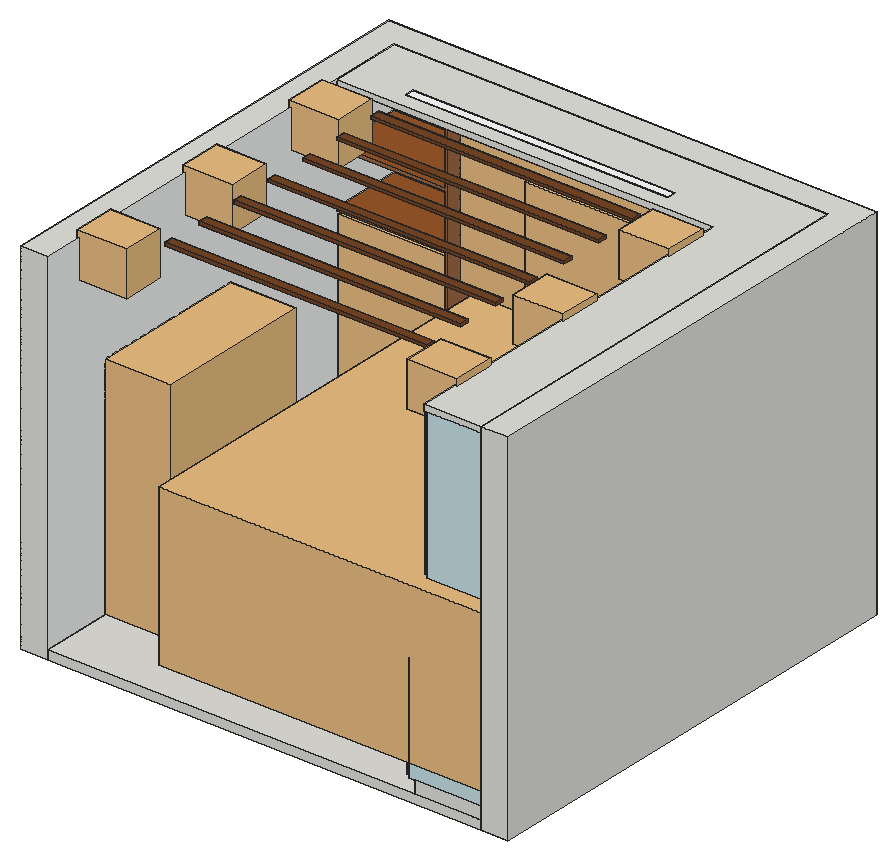
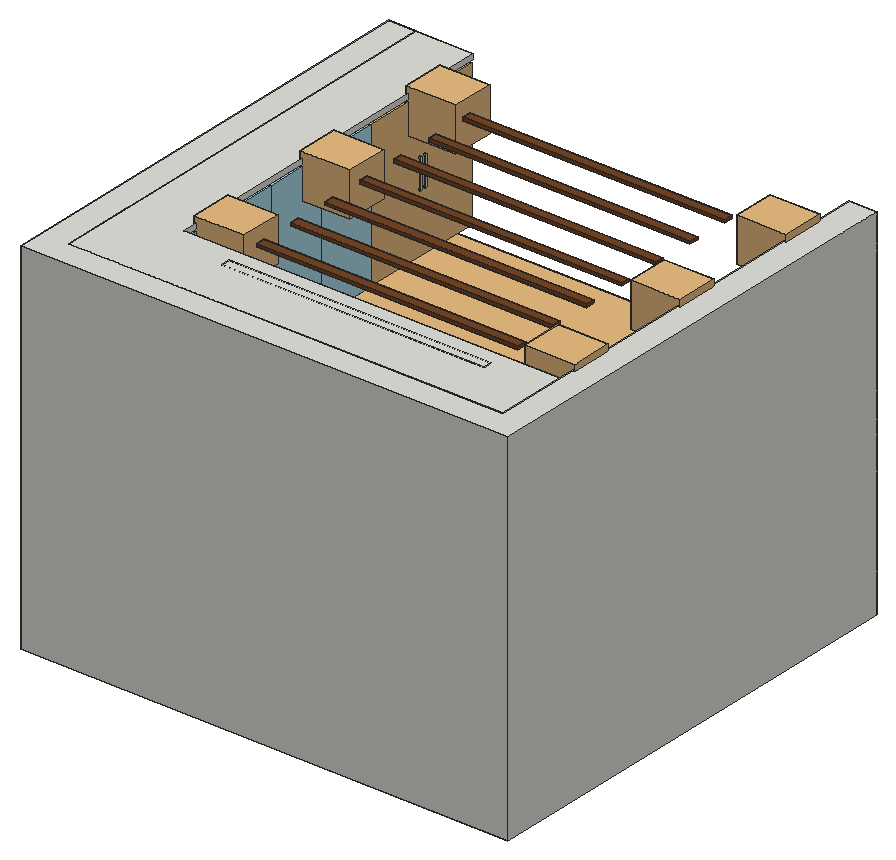
# SketchUp Ruby script. Lengths in inches.
U = 1.inch
M = Sketchup.active_model
def pt(a) = Geom::Point3d.new(a.map { |v| v * U })
def face(e, loops, mat)
  f = e.add_face(loops[0].map { |a| pt(a) })
  loops[1..].each { |l| e.add_face(l.map { |a| pt(a) }).erase! }
  f.material = f.back_material = mat if mat
  f
end
# faces: each face lists its corners as indices into pts; further lists are holes
def faces(e, pts, list, mat = nil) = list.each { |f| face(e, (f[0].is_a?(Array) ? f : [f]).map { |l| l.map { |i| pts[i] } }, mat) }
# xy, xz, yz: faces in a plane at the given z, y or x. An outline is a flat list of corners, or four numbers for a rectangle; further outlines are holes
def ring(l) = l.size == 4 ? [[l[0], l[1]], [l[2], l[1]], [l[2], l[3]], [l[0], l[3]]] : l.each_slice(2).to_a
def flat(e, list, mat, &to3) = list.each { |f| face(e, (f[0].is_a?(Array) ? f : [f]).map { |l| ring(l).map { |u, v| to3.(u, v) } }, mat) }
def xy(e, z, list, mat = nil) = flat(e, list, mat) { |x, y| [x, y, z] }
def xz(e, y, list, mat = nil) = flat(e, list, mat) { |x, z| [x, y, z] }
def yz(e, x, list, mat = nil) = flat(e, list, mat) { |y, z| [x, y, z] }
def lines(e, pts, list) = list.each { |a, b| e.add_line(pt(pts[a]), pt(pts[b])) }
# prism: a flat outline (further loops are holes) pulled along v
def prism(e, loops, v, mat = nil)
  f = face(e, loops, mat); d = Geom::Vector3d.new(v.map { |x| x * U })
  f.pushpull(f.normal.samedirection?(d) ? d.length : -d.length)
end
def box(e, o, s, mat = nil) = prism(e, [[o, [o[0] + s[0], o[1], o[2]], [o[0] + s[0], o[1] + s[1], o[2]], [o[0], o[1] + s[1], o[2]]]], [0, 0, s[2]], mat)
def at(x, y, z, deg = 0) = Geom::Transformation.translation(pt([x, y, z])) * Geom::Transformation.rotation(ORIGIN, Z_AXIS, deg.degrees)
def axes(o, x, y, z) = Geom::Transformation.new([*x, 0, *y, 0, *z, 0, *pt(o).to_a, 1])
def part(name) = M.definitions.add(name)
# library, detail: a bought-in or finely detailed component or shape, given as its bounding box
def library(name, o, s) = part(name).tap { |d| box(d.entities, o, s) }
def detail(e, o, s) = box(e.add_group.entities, o, s)
def put(e, d, t, mat = nil) = e.add_instance(d, t).tap { |i| i.material = mat if mat }
def group(e, t, mat = nil) = e.add_group.tap { |g| g.transformation = t; g.material = mat if mat }.entities
root = M.entities
M.materials.add("0184 AP 7363 HIGH SPIRITS").color = [199, 226, 231]
M.materials.add("0441 AP 9210 SOFT BLUE").color = [171, 218, 233]
M.materials.add("Dado").color = [252, 229, 201]
M.materials.add("W146Z460B75_NILAYA CITY GLAM 32611 ROLL B75").color = [241, 242, 243]
M.materials.add("[Carrera Marble]").color = [207, 207, 207]
M.materials.add("[Color M00]").color = [255, 255, 255]
M.materials.add("[Marble Carrara Gold Floor Tile]").color = [225, 223, 217]
M.materials.add("[Stone Marble]").color = [143, 138, 136]
M.materials.add("[Translucent Glass Blue]").color = [154, 179, 222]
M.materials["[Translucent Glass Blue]"].alpha = 0.5
M.materials.add("[Wood Cherry Original]").color = [152, 86, 42]
M.materials.add("[Wood Floor Parquet]").color = [160, 112, 68]
M.materials.add("[Wood Veneer 01]").color = [160, 105, 68]
M.materials.add("[Wood Veneer 01]1").color = [120, 70, 37]
c1 = library("Group\#91",[0,-4,0],[52,76,21.875])
c2 = library("French door refrigerator",[0,0,0],[35.5,29.25,69.5])
c3 = part("1")
detail(c3.entities,[-0.45,-1,-0.3],[35.9,1,11.43])
c4 = part("2")
box(c4.entities,[-1,-0.3,-0.3],[1,40.1,17.1])
c5 = library("Group\#27",[-1,-0.3,-0.3],[1,40.1,34.6])
c6 = library("Group\#7",[0,0,-31.45],[107,144,53.06])
c7 = part("3")
box(c7.entities,[-20,0,0],[20,41,0.39])
c8 = part("POI-E1497-320-1917\#1")
xy(c8.entities,0,[[0,0,0.29,0.83],[7.21,0,7.5,0.83]])
xy(c8.entities,0.64,[[0.29,0.21,7.21,0.62]])
xy(c8.entities,0.875,[[0,0.21,7.5,0.62]])
xz(c8.entities,0.21,[[0,0.64,7.5,0.875]])
xz(c8.entities,0.62,[[0,0.64,7.5,0.875]])
yz(c8.entities,0,[[0,0,0.21,0.64,0.21,0.875,0.62,0.875,0.62,0.64,0.83,0]])
yz(c8.entities,0.29,[[0,0,0.83,0,0.62,0.64,0.21,0.64]])
yz(c8.entities,7.21,[[0,0,0.21,0.64,0.62,0.64,0.83,0]])
yz(c8.entities,7.5,[[0,0,0.83,0,0.62,0.64,0.62,0.875,0.21,0.875,0.21,0.64]])
p = [[0,0.21,0.64],[0,0,0],[0.29,0,0],[0.29,0.21,0.64],[7.21,0.21,0.64],[7.21,0,0],
  [7.5,0,0],[7.5,0.21,0.64],[0,0.83,0],[0,0.62,0.64],[0.29,0.62,0.64],[0.29,0.83,0],
  [7.5,0.83,0],[7.5,0.62,0.64],[7.21,0.62,0.64],[7.21,0.83,0]]
faces(c8.entities,p,[[0,1,2,3],[4,5,6,7],[8,9,10,11],[12,13,14,15]])
c9 = library("13",[0,-0.4,-0.4],[1.79,16.97,40.8])
c10 = library("kitchen utensil",[-39.88,-27.4,0],[79.77,28.4,32.96])
c11 = library("Group\#26",[0,0,0],[28.9375,18.36,1.53])
c12 = library("Cookware hanging rail",[-2.09,-19.1875,0],[25.71,19.1875,6.07])
c13 = library("switch board",[0,0,0],[0.88,10.49,5.27])
c14 = part("6")
box(c14.entities,[-1,20.47,-0.3],[1,20.66,48.01])
box(c14.entities,[-1,-0.3,-0.3],[1,20.67,48.01])
p = [[0,20.47,47.71],[0,20.37,47.71]]
lines(c14.entities,p,[[0,1]])
c15 = part("7")
prism(c15.entities,[[[0,0.25,0],[0,0.5,0],[0.88,0.5,0],[0.88,0.25,0],[0.86,0.22,0],[0.84,0.19,0],[0.81,0.17,0],[0.79,0.14,0],[0.76,0.12,0],[0.74,0.1,0],[0.71,0.08,0],[0.68,0.06,0],[0.64,0.04,0],[0.61,0.03,0],[0.58,0.02,0],[0.54,0.01,0],[0.51,0,0],[0.47,0,0],[0.4375,0,0],[0.4,0,0],[0.37,0,0],[0.33,0.01,0],[0.3,0.02,0],[0.27,0.03,0],[0.23,0.04,0],[0.2,0.06,0],[0.17,0.08,0],[0.14,0.1,0],[0.11,0.12,0],[0.09,0.14,0],[0.0625,0.17,0],[0.04,0.19,0],[0.02,0.22,0]]],[0,0,47.41])
c16 = library("Group\#12",[0,0,0],[107,19,49.41])
c17 = library("Group\#10",[-1,-0.3,-0.3],[1,40.1,34.6])
c18 = library("Rangemaaster flat hood",[-3.82,0.71,0],[43.23,19.01,40.35])
c19 = part("Group156\#1")
p = [[0,0,0],[0,0,-10.12],[-5.02,0,-10.12],[32.7,-0.05,0],[-32.7,-0.05,0],[32.7,0.05,0],
  [32.7,0,0],[-32.7,0.05,0],[5.02,0,-10.12],[-32.7,0,0],[0,0,-16.375]]
lines(c19.entities,p,[[0,1],[1,2],[3,4],[5,6],[7,5],[1,8],[9,0],[0,6],[8,10],[4,9],[6,3],[2,10],
  [9,7]])
c20 = part("Rectangle Light")
put(c20.entities,c19,at(0,0,0))
c21 = part("5")
xy(c21.entities,-0.61,[[-17,0.0625,-16,40.83]])
xy(c21.entities,-0.44,[[-16.3125,0.0625,-16,40.83]])
xy(c21.entities,-0.11,[[-16.3125,0.0625,-16,40.83]])
xy(c21.entities,0,[[-16,0,0,40.83]],"[Translucent Glass Blue]")
xy(c21.entities,0.39,[[-17,0.0625,-16,40.83]])
xy(c21.entities,0.39,[[-16,0,0,40.83]],"[Translucent Glass Blue]")
xz(c21.entities,0,[[-16,0,0,0.39]],"[Translucent Glass Blue]")
xz(c21.entities,0.0625,[[-17,-0.61,-16,-0.61,-16,-0.44,-16.3125,-0.44,-16.3125,-0.11,-16,-0.11,-16,0.39,-17,0.39]])
xz(c21.entities,40.83,[[-16,0,0,0.39]],"[Translucent Glass Blue]")
yz(c21.entities,-17,[[0.0625,-0.61,40.83,0.39]])
yz(c21.entities,-16.3125,[[0.0625,-0.44,40.83,-0.11]])
yz(c21.entities,-16,[[0.0625,-0.61,40.83,-0.44],[0.0625,-0.11,40.83,0],[0.0625,0,40.83,0.39]])
yz(c21.entities,-16,[[0,0,0.0625,0.39]],"[Translucent Glass Blue]")
yz(c21.entities,0,[[0,0,40.83,0.39]],"[Translucent Glass Blue]")
put(c21.entities,c20,axes([-16.03,20.45,-0.19],[0,0.62341,0],[-0.20108,0,-0.97958],[-0.97958,0,0.20108]))
g1 = group(c21.entities,at(-16.3125,0.0625,-0.27))
box(g1,[0,0,0],[0.25,40.77,0.17])
c22 = library("9",[-6.9,-3.96,-12.62],[16.56,13.95,14.65])
c23 = part("11")
box(c23.entities,[-1,0,-1],[87,3,1])
xy(root,0,[[0,0,0,153,162,153,162,0,153,0,153,144,9,144,9,0]])
xy(root,3,[[131,0,153,128],[9,120,9,144,153,144,153,128,46,128,46,120]])
xy(root,7,[[131,0,153,128],[9,120,45,144],[45,120,46,144],[46,128,153,144]])
xy(root,60.16,[[153,109.21,153.5,119.7]],"[Carrera Marble]")
xy(root,65.43,[[153,109.21,153.5,119.7]],"[Carrera Marble]")
xy(root,81,[[9,120,45,143.92]],"[Wood Cherry Original]")
xy(root,82,[[9,120,45,143.92]],"[Wood Cherry Original]")
xy(root,99.5,[[9,120,45,143.92]],"[Wood Cherry Original]")
xy(root,100.5,[[9,120,45,143.92]],"[Wood Cherry Original]")
xy(root,118.03,[[134,0,153,120],[9,120,45,143.92],[45,120,46,144],[46,120,153,144]])
xy(root,120,[[0,0,9,0,9,144,153,144,153,0,162,0,162,153,0,153],[134,0,153,0,153,144,9,144,9,120,134,120]])
xz(root,0,[[0,0,9,120],[153,0,162,120],[131,3,153,7],[134,118.03,153,120]])
xz(root,109.21,[[153,60.16,153.5,65.43]],"[Carrera Marble]")
xz(root,119.7,[[153,60.16,153.5,65.43]],"[Carrera Marble]")
xz(root,120,[[9,118.03,134,120]])
xz(root,120,[[9,3,46,7]],"[Carrera Marble]")
xz(root,120,[[45,7,46,7,46,118.03,45,118.03,45,100.5,9,100.5,9,99.5,45,99.5,45,82,9,82,9,81,45,81]],"[Wood Veneer 01]")
xz(root,128,[[131,3,153,7]])
xz(root,128,[[46,3,131,7]],"[Carrera Marble]")
xz(root,143.92,[[9,81,45,82],[9,99.5,45,100.5]],"[Wood Cherry Original]")
xz(root,143.92,[[9,82,45,99.5],[9,100.5,45,118.03]],"[Wood Veneer 01]")
xz(root,144,[[9,0,153,0,153,45,46,45,46,68.62,62.64,68.62,62.64,72.3125,118.36,72.3125,118.36,68.62,153,68.62,153,120,9,120],[9,3,153,7],[45,7,46,7,46,118.03,45,118.03,45,98.5,9,98.5,9,97.5,45,97.5]])
xz(root,144,[[46,45,153,45,153,68.62,118.36,68.62,118.36,72.3125,62.64,72.3125,62.64,68.62,46,68.62]],"[Carrera Marble]")
xz(root,144,[[9,98.5,45,118.03]],"[Wood Veneer 01]")
xz(root,153,[[0,0,162,120]])
yz(root,0,[[0,0,153,120]])
yz(root,9,[[120,3,144,7],[120,81,143.92,82],[143.92,97.5,144,98.5],[120,99.5,143.92,100.5],[120,118.03,144,120]])
yz(root,9,[[0,0,144,120]],"W146Z460B75_NILAYA CITY GLAM 32611 ROLL B75")
yz(root,9,[[143.92,76,144,97.5],[143.92,98.5,144,118.03]],"[Wood Veneer 01]")
yz(root,45,[[120,7,120,81,143.92,81,143.92,76,144,76,144,7]],"[Wood Cherry Original]")
yz(root,45,[[143.92,76,144,97.5],[120,82,143.92,99.5],[143.92,98.5,144,118.03],[120,100.5,143.92,118.03]],"[Wood Veneer 01]")
yz(root,46,[[120,3,128,7]],"[Carrera Marble]")
yz(root,46,[[120,7,144,118.03]],"[Wood Veneer 01]")
yz(root,131,[[0,3,128,7]],"[Carrera Marble]")
yz(root,134,[[0,118.03,120,120]])
yz(root,153,[[0,0,144,45],[0,3,128,7],[128,3,144,7],[0,68.62,144,120],[120,118.03,144,120]])
yz(root,153,[[[0,45,144,68.62],[109.21,60.16,119.7,65.43]]],"[Carrera Marble]")
yz(root,153.5,[[109.21,60.16,119.7,65.43]],"[Carrera Marble]")
yz(root,162,[[0,0,153,120]])
p = [[153,144,45],[153,144,70.59],[9,144,76],[9,144,7]]
lines(root,p,[[0,1],[2,3]])
g2 = group(root,at(9,0,0))
xy(g2,0,[[0,0,144,144]])
xy(g2,3,[[122,0,144,0,144,144,0,144,0,120,37,120,37,128,122,128]])
xy(g2,3,[[0,0,122,0,122,128,37,128,37,120,0,120]],"[Marble Carrara Gold Floor Tile]")
xz(g2,0,[[0,0,144,3]])
xz(g2,144,[[0,0,144,3]])
yz(g2,0,[[0,0,144,3]])
yz(g2,144,[[0,0,144,3]])
put(root,c1,axes([9,24,7],[0,1,0],[0,0,1],[1,0,0]))
g3 = group(root,at(46,144,7),"0184 AP 7363 HIGH SPIRITS")
xy(g3,0,[[0,-20,83,0]])
xy(g3,1,[[1,-20,36,-1],[37,-20,67,-1],[68,-20,80,-1]])
xy(g3,11.83,[[1,-20,36,-1]])
xy(g3,12.83,[[1,-20,36,-1]])
xy(g3,17.5,[[68,-20,80,-1]])
xy(g3,18.5,[[68,-20,80,-1]])
xy(g3,23.17,[[1,-20,36,-1]])
xy(g3,24.17,[[1,-20,36,-1]])
xy(g3,35,[[1,-20,36,-1],[37,-20,67,-1],[68,-20,80,-1]])
xy(g3,36,[[0,-20,83,0]])
xz(g3,-20,[[[0,0,83,36],[37,1,67,35],[1,1,36,11.83],[1,24.17,36,35],[1,12.83,36,23.17],[68,18.5,80,35],[68,1,80,17.5]]])
xz(g3,-1,[[1,1,36,11.83],[37,1,67,35],[68,1,80,17.5],[1,12.83,36,23.17],[68,18.5,80,35],
  [1,24.17,36,35]])
xz(g3,0,[[0,0,83,36]])
yz(g3,0,[[-20,0,0,36]])
yz(g3,1,[[-20,1,-1,11.83],[-20,12.83,-1,23.17],[-20,24.17,-1,35]])
yz(g3,36,[[-20,1,-1,11.83],[-20,12.83,-1,23.17],[-20,24.17,-1,35]])
yz(g3,37,[[-20,1,-1,35]])
yz(g3,67,[[-20,1,-1,35]])
yz(g3,68,[[-20,1,-1,17.5],[-20,18.5,-1,35]])
yz(g3,80,[[-20,1,-1,17.5],[-20,18.5,-1,35]])
yz(g3,83,[[-20,0,0,36]])
g4 = group(root,at(153,0,7),"0184 AP 7363 HIGH SPIRITS")
xy(g4,0,[[-24,0,0,128],[-24,128,0,144]])
xy(g4,1,[[-24,1,-2.77,42],[-24,43,-2.77,82.5],[-24,83.5,-2.77,83.5,-2.77,143,-23.08,143,-23.08,122,-24,122]])
xy(g4,11.83,[[-23.08,83.5,-2.77,143]])
xy(g4,12.83,[[-23.08,83.5,-2.77,143]])
xy(g4,17.5,[[-24,43,-2.77,82.5]])
xy(g4,18.5,[[-24,43,-2.77,82.5]])
xy(g4,23.17,[[-23.08,83.5,-2.77,143]])
xy(g4,24.17,[[-23.08,83.5,-2.77,143]])
xy(g4,30.3125,[[-22,43,-5.47,43,-5.47,79.65,-22,79.57]])
xy(g4,33.0625,[[-22,42.27,-5.47,42.35,-5.47,43,-22,43],[-24,43,-24,82.5,-2.77,82.5,-2.77,43,-5.47,43,-5.47,79.65,-22,79.57,-22,43]])
xy(g4,35,[[-24,1,-2.77,42],[-24,83.5,-24,122,-23.08,122,-23.08,143,-2.77,143,-2.77,83.5]])
xy(g4,36,[[[-24,0,0,144],[-22,42.27,-22,80.625,-5.47,80.71,-5.47,42.35]]])
xz(g4,0,[[-24,0,0,36]])
xz(g4,1,[[-24,1,-2.77,35]])
xz(g4,42,[[-24,1,-2.77,35]])
xz(g4,43,[[-24,1,-2.77,17.5],[-24,18.5,-24,33.0625,-22,33.0625,-22,30.3125,-5.47,30.3125,-5.47,33.0625,-2.77,33.0625,-2.77,18.5],[-22,30.3125,-5.47,33.0625]])
xz(g4,82.5,[[-24,1,-2.77,17.5],[-24,18.5,-2.77,33.0625]])
xz(g4,83.5,[[-24,1,-24,35,-2.77,35,-2.77,24.17,-23.08,24.17,-23.08,23.17,-2.77,23.17,-2.77,12.83,-23.08,12.83,-23.08,11.83,-2.77,11.83,-2.77,1]])
xz(g4,122,[[-24,1,-23.08,35]])
xz(g4,143,[[-24,1,-23.08,35],[-2.77,1,-1.85,1,-1.85,35,-2.77,35,-2.77,24.17,-23.08,24.17,-23.08,23.17,-2.77,23.17,-2.77,12.83,-23.08,12.83,-23.08,11.83,-2.77,11.83],[-23.08,1,-2.77,11.83],[-23.08,12.83,-2.77,23.17],[-23.08,24.17,-2.77,35]])
xz(g4,144,[[-24,0,0,36]])
yz(g4,-24,[[[0,0,144,36],[1,1,42,35],[83.5,1,122,35],[43,1,82.5,17.5],[124,1,143,35],[43,18.5,82.5,33.0625]]])
yz(g4,-23.08,[[122,1,143,11.83],[83.5,11.83,122,12.83],[122,11.83,143,12.83],[122,12.83,143,23.17],[83.5,23.17,122,24.17],
  [122,23.17,143,24.17],[122,24.17,143,35]])
yz(g4,-22,[[43,30.3125,79.57,33.0625],[42.27,33.0625,79.57,33.0625,80.625,36,42.27,36]])
yz(g4,-5.47,[[43,30.3125,79.65,33.0625],[42.35,33.0625,42.35,36,80.71,36,79.65,33.0625]])
yz(g4,-2.77,[[1,1,42,35],[43,1,82.5,17.5],[83.5,1,143,11.83],[83.5,12.83,143,23.17],[43,18.5,82.5,33.0625],
  [83.5,24.17,143,35]])
yz(g4,-1.85,[[43,1,143,35]])
yz(g4,0,[[0,0,144,36]])
p = [[-5.47,79.65,33.0625],[-22,79.57,33.0625],[-22,79.57,30.3125],[-5.47,79.65,30.3125],[-22,42.27,36],[-5.47,42.35,36],
  [-5.47,42.35,33.0625],[-22,42.27,33.0625],[-5.47,80.71,36],[-22,80.625,36],[-24,124,1],[-23.08,124,1],
  [-24,124,35],[-23.08,124,35],[-2.77,43,35],[-1.85,43,35],[-2.77,43,1],[-1.85,43,1]]
faces(g4,p,[[0,1,2,3],[4,5,6,7],[8,9,1,0]])
lines(g4,p,[[10,11],[12,13],[14,15],[16,17]])
put(root,c2,axes([45,149.25,7],[-1,0,0],[0,-1,0],[0,0,1.05223]))
put(root,c3,at(47,124,8),"0441 AP 9210 SOFT BLUE")
put(root,c4,at(129,43,8),"0441 AP 9210 SOFT BLUE")
g5 = group(root,at(83,124,8),"0441 AP 9210 SOFT BLUE")
box(g5,[-0.5,-1,-0.3],[31,1,34.6])
g6 = group(root,at(114,124,8),"0441 AP 9210 SOFT BLUE")
box(g6,[-0.45,-1,17.05],[13.9,1,17.25])
box(g6,[-0.45,-1,-0.3],[13.9,1,17.25])
g7 = group(root,at(129,83.5,8),"0441 AP 9210 SOFT BLUE")
box(g7,[-1,-0.3,-0.3],[1,39.1,34.6])
put(root,c5,axes([129,1,8],[1,0,0],[0,1.04,0],[0,0,1]),"0441 AP 9210 SOFT BLUE")
put(root,c6,at(46,0,43),"[Stone Marble]")
put(root,c7,at(150,1,19.2),"[Translucent Glass Blue]")
put(root,c3,axes([47,124,19.83],[1,0,0],[0,1,0],[0,0,0.95385]),"0441 AP 9210 SOFT BLUE")
put(root,c8,axes([128,22.08,22.14],[0,0,1],[0,1,0],[-1,0,0]))
put(root,c8,axes([128,20.92,22.14],[0,0,1],[0,-1,0],[-1,0,0]))
put(root,c4,at(129,43,25.5),"0441 AP 9210 SOFT BLUE")
put(root,c7,at(150,1,30.4),"[Translucent Glass Blue]")
put(root,c3,at(47,124,31.17),"0441 AP 9210 SOFT BLUE")
put(root,c9,at(29,25,38),"[Wood Veneer 01]1")
put(root,c9,at(29,58.83,38),"[Wood Veneer 01]1")
put(root,c9,axes([29,42.17,38],[1,0,0],[0,0.96907,0],[0,0,1]),"[Wood Veneer 01]1")
put(root,c10,axes([136.65,143.59,45],[0.41,0,0],[0,0.41,0],[0,0,0.41]))
put(root,c11,at(76.6875,123.1,45))
put(root,c12,axes([51.26,144,66.375],[1,0,0],[0,0,1],[0,-1,0]))
put(root,c13,at(153.29,119.7,60.16,180))
g8 = group(root,at(46,0,68.62),"0184 AP 7363 HIGH SPIRITS")
put(g8,c14,axes([89,42.83,1],[1,0,0],[0,0.98776,0],[0,0,1]),"0441 AP 9210 SOFT BLUE")
put(g8,c14,at(89,84.17,1),"0441 AP 9210 SOFT BLUE")
put(g8,c15,at(0.83,142.5,1),"[Wood Floor Parquet]")
put(g8,c15,at(1.77,142.5,1),"[Wood Floor Parquet]")
put(g8,c15,at(2.71,142.5,1),"[Wood Floor Parquet]")
put(g8,c15,at(3.65,142.5,1),"[Wood Floor Parquet]")
put(g8,c15,at(4.59,142.5,1),"[Wood Floor Parquet]")
put(g8,c15,at(5.53,142.5,1),"[Wood Floor Parquet]")
put(g8,c15,at(6.47,142.5,1),"[Wood Floor Parquet]")
put(g8,c15,at(7.41,142.5,1),"[Wood Floor Parquet]")
put(g8,c15,at(8.35,142.5,1),"[Wood Floor Parquet]")
put(g8,c15,at(9.29,142.5,1),"[Wood Floor Parquet]")
put(g8,c15,at(10.23,142.5,1),"[Wood Floor Parquet]")
put(g8,c15,at(11.17,142.5,1),"[Wood Floor Parquet]")
put(g8,c15,at(12.11,142.5,1),"[Wood Floor Parquet]")
put(g8,c15,at(13.05,142.5,1),"[Wood Floor Parquet]")
put(g8,c15,at(13.99,142.5,1),"[Wood Floor Parquet]")
put(g8,c15,at(14.93,142.5,1),"[Wood Floor Parquet]")
put(g8,c15,at(77.89,142.5,1),"[Wood Floor Parquet]")
put(g8,c15,at(79.77,142.5,1),"[Wood Floor Parquet]")
put(g8,c15,at(74.14,142.5,1),"[Wood Floor Parquet]")
put(g8,c15,at(78.83,142.5,1),"[Wood Floor Parquet]")
put(g8,c15,at(80.71,142.5,1),"[Wood Floor Parquet]")
put(g8,c15,at(75.08,142.5,1),"[Wood Floor Parquet]")
put(g8,c15,at(76.95,142.5,1),"[Wood Floor Parquet]")
put(g8,c15,at(81.65,142.5,1),"[Wood Floor Parquet]")
put(g8,c15,at(76.02,142.5,1),"[Wood Floor Parquet]")
put(g8,c15,at(73.2,142.5,1),"[Wood Floor Parquet]")
put(g8,c15,at(86.35,142.5,1),"[Wood Floor Parquet]")
put(g8,c15,at(84.47,142.5,1),"[Wood Floor Parquet]")
put(g8,c15,at(85.41,142.5,1),"[Wood Floor Parquet]")
put(g8,c15,at(83.53,142.5,1),"[Wood Floor Parquet]")
put(g8,c15,at(82.59,142.5,1),"[Wood Floor Parquet]")
put(g8,c15,at(87.29,142.5,1),"[Wood Floor Parquet]")
g9 = group(g8,at(107,0,0))
xy(g9,0,[[-18,0,-18,143.5,-0.5,143.5,-0.5,2,0,2,0,0]])
xy(g9,0.5,[[-0.5,2,-0.5,143.5,-18,143.5,-18,144,0,144,0,2]])
xy(g9,1,[[-18,1,-1,41.83],[-18,42.83,-1,83.17],[-18,84.17,-1,84.17,-1,142,-18,142,-18,126,-17,126,-17,125,-18,125]])
xy(g9,12.35,[[-17,42.83,-1,83.17],[-17,84.17,-1,142]])
xy(g9,13.35,[[-17,42.83,-1,83.17],[-17,84.17,-1,142]])
xy(g9,24.2,[[-17,42.83,-1,83.17],[-17,84.17,-1,142]])
xy(g9,25.2,[[-17,42.83,-1,83.17],[-17,84.17,-1,142]])
xy(g9,36.06,[[-17,42.83,-1,83.17],[-17,84.17,-1,142]])
xy(g9,37.06,[[-17,42.83,-1,83.17],[-17,84.17,-1,142]])
xy(g9,48.41,[[-18,1,-1,41.83],[-18,42.83,-1,83.17],[-18,84.17,-18,125,-17,125,-17,126,-18,126,-18,142,-1,142,-1,84.17]])
xy(g9,49.41,[[-18,0,0,144]])
xz(g9,0,[[-18,0,0,49.41]])
xz(g9,1,[[-18,1,-1,48.41]])
xz(g9,2,[[-0.5,0,0,0.5]])
xz(g9,41.83,[[-18,1,-1,48.41]])
xz(g9,42.83,[[-18,1,-18,48.41,-1,48.41,-1,37.06,-17,37.06,-17,36.06,-1,36.06,-1,25.2,-17,25.2,-17,24.2,-1,24.2,-1,13.35,-17,13.35,-17,12.35,-1,12.35,-1,1]])
xz(g9,83.17,[[-18,1,-1,1,-1,12.35,-17,12.35,-17,13.35,-1,13.35,-1,24.2,-17,24.2,-17,25.2,-1,25.2,-1,36.06,-17,36.06,-17,37.06,-1,37.06,-1,48.41,-18,48.41]])
xz(g9,84.17,[[-18,1,-18,48.41,-1,48.41,-1,37.06,-17,37.06,-17,36.06,-1,36.06,-1,25.2,-17,25.2,-17,24.2,-1,24.2,-1,13.35,-17,13.35,-17,12.35,-1,12.35,-1,1]])
xz(g9,125,[[-18,1,-17,48.41]])
xz(g9,126,[[-18,1,-17,48.41]])
xz(g9,142,[[-18,1,-1,1,-1,12.35,-17,12.35,-17,13.35,-1,13.35,-1,24.2,-17,24.2,-17,25.2,-1,25.2,-1,36.06,-17,36.06,-17,37.06,-1,37.06,-1,48.41,-18,48.41]])
xz(g9,143.5,[[-18,0,-0.5,0.5]])
xz(g9,144,[[-18,0.5,0,49.41]])
yz(g9,-18,[[[0,0,0,49.41,144,49.41,144,0.5,143.5,0.5,143.5,0],[1,1,41.83,48.41],[84.17,1,125,48.41],[42.83,1,83.17,48.41],[126,1,143,48.41]],[142,1,143,48.41]])
yz(g9,-17,[[125,1,126,12.35],[42.83,12.35,83.17,13.35],[84.17,12.35,125,13.35],[125,12.35,126,13.35],[126,12.35,142,13.35],
  [125,13.35,126,24.2],[42.83,24.2,83.17,25.2],[84.17,24.2,125,25.2],[125,24.2,126,25.2],[126,24.2,142,25.2],
  [125,25.2,126,36.06],[42.83,36.06,83.17,37.06],[84.17,36.06,125,37.06],[125,36.06,126,37.06],[126,36.06,142,37.06],
  [125,37.06,126,48.41]])
yz(g9,-1,[[1,1,41.83,48.41],[42.83,1,83.17,12.35],[84.17,1,142,12.35],[42.83,13.35,83.17,24.2],[84.17,13.35,142,24.2],
  [42.83,25.2,83.17,36.06],[84.17,25.2,142,36.06],[42.83,37.06,83.17,48.41],[84.17,37.06,142,48.41]])
yz(g9,-0.5,[[2,0,143.5,0.5]])
yz(g9,0,[[0,0,2,0.5],[0,0.5,144,49.41]])
p = [[-0.5,0,0.5],[-0.5,2,0.5]]
lines(g9,p,[[0,1]])
g10 = group(g9,at(-0.5,0,0),"Dado")
prism(g10,[[[0.5,2,0.125],[0,2,0.125],[0,143.5,0.125],[-17.5,143.5,0.125],[-17.5,144,0.125],[0.5,144,0.125]]],[0,0,0.375])
put(g8,c16,axes([0,125,0],[0.83178,0,0],[0,1,0],[0,0,1]),"0441 AP 9210 SOFT BLUE")
put(g8,c17,axes([89,1,1.12],[1,0,0],[0,1.04,0],[0,0,1.38756]))
put(root,c18,at(72.95,122.5,69))
put(root,c21,at(152,1,83.34))
put(root,c8,axes([134,22.08,89.4],[0,0,1.3189],[0,1,0],[-1,0,0]))
put(root,c8,axes([134,20.92,89.4],[0,0,1.3189],[0,-1,0],[-1,0,0]))
put(root,c21,at(152,1,95.1))
put(root,c21,at(152,1,106.85))
put(root,c22,at(125,17,120))
put(root,c22,at(125,61,120))
put(root,c22,at(125,105,120))
put(root,c22,axes([18,17,120],[-1,0,0],[0,1,0],[0,0,1]))
put(root,c22,axes([18,61,120],[-1,0,0],[0,1,0],[0,0,1]))
put(root,c22,axes([18,105,120],[-1,0,0],[0,1,0],[0,0,1]))
put(root,c23,at(29,125,120),"[Color M00]")
put(root,c23,at(29,110.71,120),"[Wood Veneer 01]1")
put(root,c23,at(29,96.43,120),"[Wood Veneer 01]1")
put(root,c23,at(29,82.14,120),"[Wood Veneer 01]1")
put(root,c23,at(29,67.86,120),"[Wood Veneer 01]1")
put(root,c23,at(29,53.57,120),"[Wood Veneer 01]1")
put(root,c23,at(29,39.29,120),"[Wood Veneer 01]1")
put(root,c23,at(29,25,120),"[Wood Veneer 01]1")
